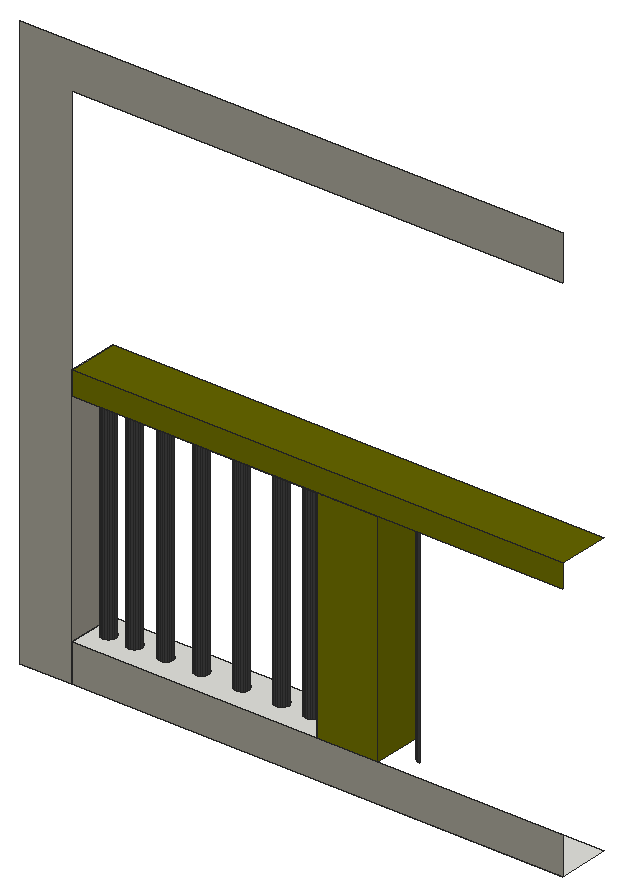
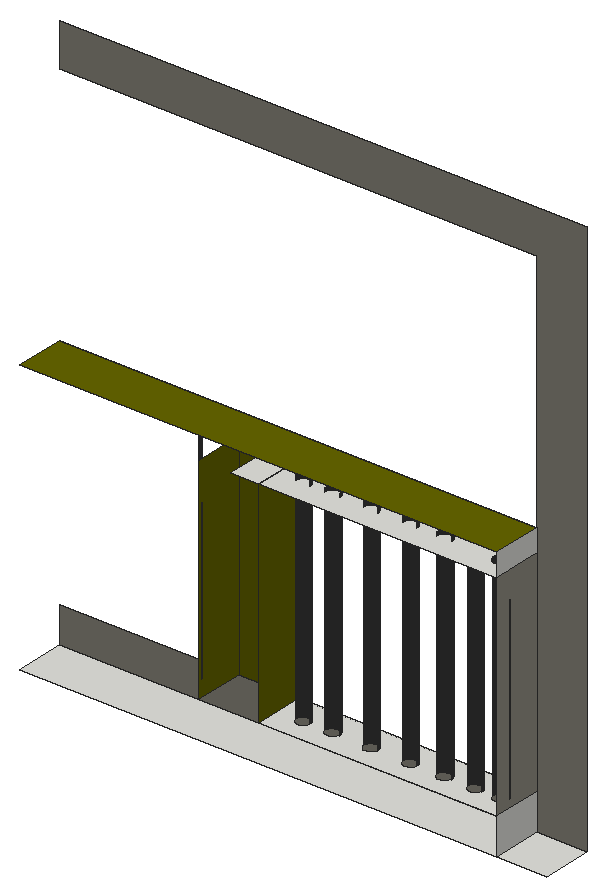
# SketchUp Ruby script. Lengths in inches.
U = 1.inch
M = Sketchup.active_model
def pt(a) = Geom::Point3d.new(a.map { |v| v * U })
def face(e, loops, mat)
  f = e.add_face(loops[0].map { |a| pt(a) })
  loops[1..].each { |l| e.add_face(l.map { |a| pt(a) }).erase! }
  f.material = f.back_material = mat if mat
  f
end
# faces: each face lists its corners as indices into pts; further lists are holes
def faces(e, pts, list, mat = nil) = list.each { |f| face(e, (f[0].is_a?(Array) ? f : [f]).map { |l| l.map { |i| pts[i] } }, mat) }
# xy, xz, yz: faces in a plane at the given z, y or x. An outline is a flat list of corners, or four numbers for a rectangle; further outlines are holes
def ring(l) = l.size == 4 ? [[l[0], l[1]], [l[2], l[1]], [l[2], l[3]], [l[0], l[3]]] : l.each_slice(2).to_a
def flat(e, list, mat, &to3) = list.each { |f| face(e, (f[0].is_a?(Array) ? f : [f]).map { |l| ring(l).map { |u, v| to3.(u, v) } }, mat) }
def xy(e, z, list, mat = nil) = flat(e, list, mat) { |x, y| [x, y, z] }
def xz(e, y, list, mat = nil) = flat(e, list, mat) { |x, z| [x, y, z] }
def yz(e, x, list, mat = nil) = flat(e, list, mat) { |y, z| [x, y, z] }
def lines(e, pts, list) = list.each { |a, b| e.add_line(pt(pts[a]), pt(pts[b])) }
# prism: a flat outline (further loops are holes) pulled along v
def prism(e, loops, v, mat = nil)
  f = face(e, loops, mat); d = Geom::Vector3d.new(v.map { |x| x * U })
  f.pushpull(f.normal.samedirection?(d) ? d.length : -d.length)
end
def box(e, o, s, mat = nil) = prism(e, [[o, [o[0] + s[0], o[1], o[2]], [o[0] + s[0], o[1] + s[1], o[2]], [o[0], o[1] + s[1], o[2]]]], [0, 0, s[2]], mat)
def at(x, y, z, deg = 0) = Geom::Transformation.translation(pt([x, y, z])) * Geom::Transformation.rotation(ORIGIN, Z_AXIS, deg.degrees)
def axes(o, x, y, z) = Geom::Transformation.new([*x, 0, *y, 0, *z, 0, *pt(o).to_a, 1])
def part(name) = M.definitions.add(name)
# library, detail: a bought-in or finely detailed component or shape, given as its bounding box
def library(name, o, s) = part(name).tap { |d| box(d.entities, o, s) }
def detail(e, o, s) = box(e.add_group.entities, o, s)
def put(e, d, t, mat = nil) = e.add_instance(d, t).tap { |i| i.material = mat if mat }
def group(e, t, mat = nil) = e.add_group.tap { |g| g.transformation = t; g.material = mat if mat }.entities
root = M.entities
M.materials.add("[Color E08]").color = [102, 102, 0]
M.materials.add("[Color M07]").color = [58, 58, 58]
M.materials.add("[Formica Graystone]").color = [149, 146, 135]
xy(root,0,[[33.03,52.46,37.72,57.16],[37.72,52.46,82.62,57.16]])
xy(root,3.4375,[[[37.72,52.46,60.17,57.16],[39.18,54.27,39,54.29,38.83,54.36,38.69,54.47,38.58,54.61,38.51,54.78,38.49,54.96,38.51,55.13,38.58,55.3,38.69,55.44,38.83,55.55,39,55.62,39.18,55.64,39.35,55.62,39.52,55.55,39.66,55.44,39.77,55.3,39.84,55.13,39.86,54.96,39.84,54.78,39.77,54.61,39.66,54.47,39.52,54.36,39.35,54.29],[57.74,54.27,57.5625,54.29,57.4,54.36,57.25,54.47,57.14,54.61,57.07,54.78,57.05,54.96,57.07,55.13,57.14,55.3,57.25,55.44,57.4,55.55,57.5625,55.62,57.74,55.64,57.92,55.62,58.08,55.55,58.23,55.44,58.33,55.3,58.4,55.13,58.43,54.96,58.4,54.78,58.33,54.61,58.23,54.47,58.08,54.36,57.92,54.29],[41.55,54.27,41.375,54.29,41.21,54.36,41.07,54.47,40.96,54.61,40.89,54.78,40.86,54.96,40.89,55.13,40.96,55.3,41.07,55.44,41.21,55.55,41.375,55.62,41.55,55.64,41.73,55.62,41.9,55.55,42.04,55.44,42.15,55.3,42.22,55.13,42.24,54.96,42.22,54.78,42.15,54.61,42.04,54.47,41.9,54.36,41.73,54.29],[54.99,54.27,54.8125,54.29,54.65,54.36,54.5,54.47,54.39,54.61,54.32,54.78,54.3,54.96,54.32,55.13,54.39,55.3,54.5,55.44,54.65,55.55,54.8125,55.62,54.99,55.64,55.17,55.62,55.33,55.55,55.48,55.44,55.58,55.3,55.65,55.13,55.68,54.96,55.65,54.78,55.58,54.61,55.48,54.47,55.33,54.36,55.17,54.29],[44.43,54.27,44.25,54.29,44.08,54.36,43.94,54.47,43.83,54.61,43.76,54.78,43.74,54.96,43.76,55.13,43.83,55.3,43.94,55.44,44.08,55.55,44.25,55.62,44.43,55.64,44.6,55.62,44.77,55.55,44.91,55.44,45.02,55.3,45.09,55.13,45.11,54.96,45.09,54.78,45.02,54.61,44.91,54.47,44.77,54.36,44.6,54.29],[51.36,54.27,51.1875,54.29,51.02,54.36,50.88,54.47,50.77,54.61,50.7,54.78,50.68,54.96,50.7,55.13,50.77,55.3,50.88,55.44,51.02,55.55,51.1875,55.62,51.36,55.64,51.54,55.62,51.71,55.55,51.85,55.44,51.96,55.3,52.03,55.13,52.05,54.96,52.03,54.78,51.96,54.61,51.85,54.47,51.71,54.36,51.54,54.29],[47.68,54.27,47.5,54.29,47.33,54.36,47.19,54.47,47.08,54.61,47.01,54.78,46.99,54.96,47.01,55.13,47.08,55.3,47.19,55.44,47.33,55.55,47.5,55.62,47.68,55.64,47.85,55.62,48.02,55.55,48.16,55.44,48.27,55.3,48.34,55.13,48.36,54.96,48.34,54.78,48.27,54.61,48.16,54.47,48.02,54.36,47.85,54.29]]])
xy(root,23.55,[[[37.72,52.46,60.17,57.16],[39.18,54.27,39.35,54.29,39.52,54.36,39.66,54.47,39.77,54.61,39.84,54.78,39.86,54.96,39.84,55.13,39.77,55.3,39.66,55.44,39.52,55.55,39.35,55.62,39.18,55.64,39,55.62,38.83,55.55,38.69,55.44,38.58,55.3,38.51,55.13,38.49,54.96,38.51,54.78,38.58,54.61,38.69,54.47,38.83,54.36,39,54.29]],[60.17,52.46,62.79,57.16]])
xy(root,25.6875,[[37.72,52.46,82.62,57.16]],"[Color E08]")
xz(root,52.46,[[60.17,3.4375,65.76,23.55],[37.72,23.55,82.62,25.6875]],"[Color E08]")
xz(root,52.46,[[33.03,0,37.72,0,37.72,48.59,82.62,48.59,82.62,52.6875,33.03,52.6875],[37.72,0,82.62,3.4375]],"[Formica Graystone]")
yz(root,37.72,[[52.46,0,57.16,3.4375],[52.46,23.55,57.16,25.6875]])
yz(root,37.72,[[52.46,3.4375,57.16,23.55]],"[Formica Graystone]")
yz(root,60.17,[[52.46,3.4375,57.16,23.55]],"[Color E08]")
yz(root,65.76,[[52.46,3.4375,57.16,23.55]],"[Color E08]")
p = [[38.83,54.36,3.4375],[39,54.29,3.4375],[39,54.29,23.55],[38.83,54.36,23.55],[39.18,54.27,3.4375],[39.18,54.27,23.55],
  [39.35,54.29,3.4375],[39.35,54.29,23.55],[39.52,54.36,3.4375],[39.52,54.36,23.55],[41.21,54.36,3.4375],[41.375,54.29,3.4375],
  [41.375,54.29,22.875],[41.21,54.36,22.875],[41.55,54.27,3.4375],[41.55,54.27,22.875],[41.73,54.29,3.4375],[41.73,54.29,22.875],
  [41.9,54.36,3.4375],[41.9,54.36,22.875],[44.08,54.36,3.4375],[44.25,54.29,3.4375],[44.25,54.29,23.875],[44.08,54.36,23.875],
  [44.43,54.27,3.4375],[44.43,54.27,23.875],[44.6,54.29,3.4375],[44.6,54.29,23.875],[44.77,54.36,3.4375],[44.77,54.36,23.875],
  [47.33,54.36,3.4375],[47.5,54.29,3.4375],[47.5,54.29,23.9375],[47.33,54.36,23.9375],[47.68,54.27,3.4375],[47.68,54.27,23.9375],
  [47.85,54.29,3.4375],[47.85,54.29,23.9375],[48.02,54.36,3.4375],[48.02,54.36,23.9375],[51.02,54.36,3.4375],[51.1875,54.29,3.4375],
  [51.1875,54.29,23.9375],[51.02,54.36,23.9375],[51.36,54.27,3.4375],[51.36,54.27,23.9375],[51.54,54.29,3.4375],[51.54,54.29,23.9375],
  [51.71,54.36,3.4375],[51.71,54.36,23.9375],[54.65,54.36,3.4375],[54.8125,54.29,3.4375],[54.8125,54.29,23.8125],[54.65,54.36,23.8125],
  [54.99,54.27,3.4375],[54.99,54.27,23.8125],[55.17,54.29,3.4375],[55.17,54.29,23.8125],[55.33,54.36,3.4375],[55.33,54.36,23.8125],
  [57.4,54.36,3.4375],[57.5625,54.29,3.4375],[57.5625,54.29,23.9375],[57.4,54.36,23.9375],[57.74,54.27,3.4375],[57.74,54.27,23.9375],
  [57.92,54.29,3.4375],[57.92,54.29,23.9375],[58.08,54.36,3.4375],[58.08,54.36,23.9375],[67.77,54.36,3.4375],[67.9375,54.29,3.4375],
  [67.9375,54.29,25.0625],[67.77,54.36,25.0625],[68.11,54.27,3.4375],[68.11,54.27,25.0625],[38.69,54.47,3.4375],[38.69,54.47,23.55],
  [39.66,54.47,3.4375],[39.66,54.47,23.55],[41.07,54.47,3.4375],[41.07,54.47,22.875],[42.04,54.47,3.4375],[42.04,54.47,22.875],
  [43.94,54.47,3.4375],[43.94,54.47,23.875],[44.91,54.47,3.4375],[44.91,54.47,23.875],[47.19,54.47,3.4375],[47.19,54.47,23.9375],
  [48.16,54.47,3.4375],[48.16,54.47,23.9375],[50.88,54.47,3.4375],[50.88,54.47,23.9375],[51.85,54.47,3.4375],[51.85,54.47,23.9375],
  [54.5,54.47,3.4375],[54.5,54.47,23.8125],[55.48,54.47,3.4375],[55.48,54.47,23.8125],[57.25,54.47,3.4375],[57.25,54.47,23.9375],
  [58.23,54.47,3.4375],[58.23,54.47,23.9375],[67.63,54.47,3.4375],[67.63,54.47,25.0625],[38.58,54.61,3.4375],[38.58,54.61,23.55],
  [39.77,54.61,3.4375],[39.77,54.61,23.55],[40.96,54.61,3.4375],[40.96,54.61,22.875],[42.15,54.61,3.4375],[42.15,54.61,22.875],
  [43.83,54.61,3.4375],[43.83,54.61,23.875],[45.02,54.61,3.4375],[45.02,54.61,23.875],[47.08,54.61,3.4375],[47.08,54.61,23.9375],
  [48.27,54.61,3.4375],[48.27,54.61,23.9375],[50.77,54.61,3.4375],[50.77,54.61,23.9375],[51.96,54.61,3.4375],[51.96,54.61,23.9375],
  [54.39,54.61,3.4375],[54.39,54.61,23.8125],[55.58,54.61,3.4375],[55.58,54.61,23.8125],[57.14,54.61,3.4375],[57.14,54.61,23.9375],
  [58.33,54.61,3.4375],[58.33,54.61,23.9375],[67.52,54.61,3.4375],[67.52,54.61,25.0625],[38.51,54.78,3.4375],[38.51,54.78,23.55],
  [39.84,54.78,3.4375],[39.84,54.78,23.55],[40.89,54.78,3.4375],[40.89,54.78,22.875],[42.22,54.78,3.4375],[42.22,54.78,22.875],
  [43.76,54.78,3.4375],[43.76,54.78,23.875],[45.09,54.78,3.4375],[45.09,54.78,23.875],[47.01,54.78,3.4375],[47.01,54.78,23.9375],
  [48.34,54.78,3.4375],[48.34,54.78,23.9375],[50.7,54.78,3.4375],[50.7,54.78,23.9375],[52.03,54.78,3.4375],[52.03,54.78,23.9375],
  [54.32,54.78,3.4375],[54.32,54.78,23.8125],[55.65,54.78,3.4375],[55.65,54.78,23.8125],[57.07,54.78,3.4375],[57.07,54.78,23.9375],
  [58.4,54.78,3.4375],[58.4,54.78,23.9375],[67.45,54.78,3.4375],[67.45,54.78,25.0625],[38.49,54.96,3.4375],[38.49,54.96,23.55],
  [39.86,54.96,3.4375],[39.86,54.96,23.55],[40.86,54.96,3.4375],[40.86,54.96,22.875],[42.24,54.96,3.4375],[42.24,54.96,22.875],
  [43.74,54.96,3.4375],[43.74,54.96,23.875],[45.11,54.96,3.4375],[45.11,54.96,23.875],[46.99,54.96,3.4375],[46.99,54.96,23.9375],
  [48.36,54.96,3.4375],[48.36,54.96,23.9375],[50.68,54.96,3.4375],[50.68,54.96,23.9375],[52.05,54.96,3.4375],[52.05,54.96,23.9375],
  [54.3,54.96,3.4375],[54.3,54.96,23.8125],[55.68,54.96,3.4375],[55.68,54.96,23.8125],[57.05,54.96,3.4375],[57.05,54.96,23.9375],
  [58.43,54.96,3.4375],[58.43,54.96,23.9375],[67.43,54.96,3.4375],[67.43,54.96,25.0625]]
faces(root,p,[[0,1,2,3],[1,4,5,2],[4,6,7,5],[6,8,9,7],[10,11,12,13],[11,14,15,12],[14,16,17,15],[16,18,19,17],
  [20,21,22,23],[21,24,25,22],[24,26,27,25],[26,28,29,27],[30,31,32,33],[31,34,35,32],[34,36,37,35],[36,38,39,37],
  [40,41,42,43],[41,44,45,42],[44,46,47,45],[46,48,49,47],[50,51,52,53],[51,54,55,52],[54,56,57,55],[56,58,59,57],
  [60,61,62,63],[61,64,65,62],[64,66,67,65],[66,68,69,67],[70,71,72,73],[71,74,75,72],[76,0,3,77],[8,78,79,9],
  [80,10,13,81],[18,82,83,19],[84,20,23,85],[28,86,87,29],[88,30,33,89],[38,90,91,39],[92,40,43,93],[48,94,95,49],
  [96,50,53,97],[58,98,99,59],[100,60,63,101],[68,102,103,69],[104,70,73,105],[106,76,77,107],[78,108,109,79],[110,80,81,111],
  [82,112,113,83],[114,84,85,115],[86,116,117,87],[118,88,89,119],[90,120,121,91],[122,92,93,123],[94,124,125,95],[126,96,97,127],
  [98,128,129,99],[130,100,101,131],[102,132,133,103],[134,104,105,135],[136,106,107,137],[108,138,139,109],[140,110,111,141],[112,142,143,113],
  [144,114,115,145],[116,146,147,117],[148,118,119,149],[120,150,151,121],[152,122,123,153],[124,154,155,125],[156,126,127,157],[128,158,159,129],
  [160,130,131,161],[132,162,163,133],[164,134,135,165],[166,136,137,167],[138,168,169,139],[170,140,141,171],[142,172,173,143],[174,144,145,175],
  [146,176,177,147],[178,148,149,179],[150,180,181,151],[182,152,153,183],[154,184,185,155],[186,156,157,187],[158,188,189,159],[190,160,161,191],
  [162,192,193,163],[194,164,165,195]],"[Color M07]")
